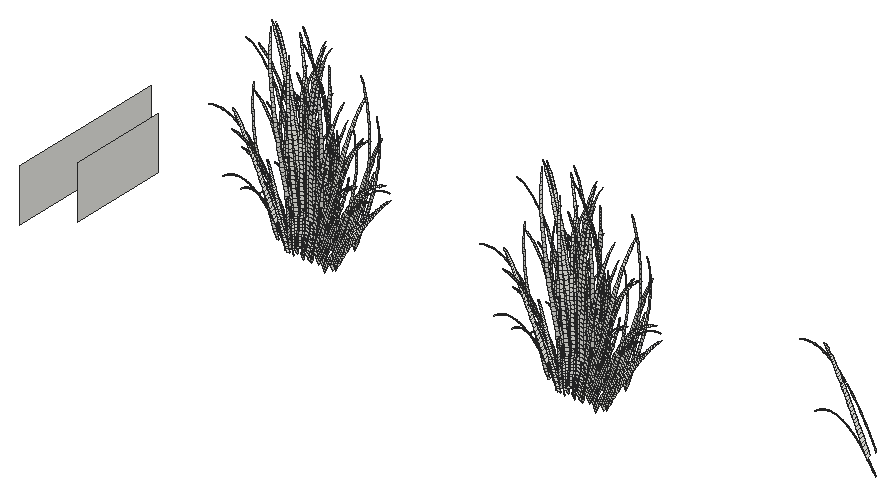
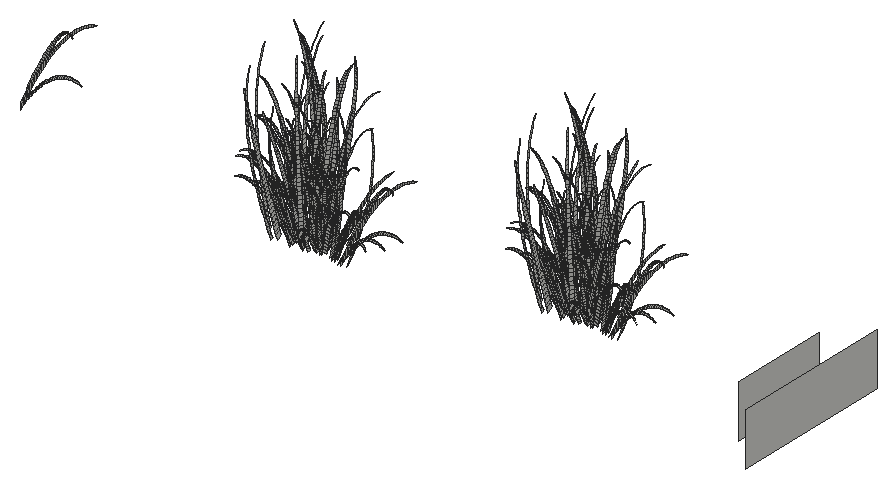
# SketchUp Ruby script. Lengths in inches.
U = 1.inch
M = Sketchup.active_model
def pt(a) = Geom::Point3d.new(a.map { |v| v * U })
def face(e, loops, mat)
  f = e.add_face(loops[0].map { |a| pt(a) })
  loops[1..].each { |l| e.add_face(l.map { |a| pt(a) }).erase! }
  f.material = f.back_material = mat if mat
  f
end
# faces: each face lists its corners as indices into pts; further lists are holes
def faces(e, pts, list, mat = nil) = list.each { |f| face(e, (f[0].is_a?(Array) ? f : [f]).map { |l| l.map { |i| pts[i] } }, mat) }
# xy, xz, yz: faces in a plane at the given z, y or x. An outline is a flat list of corners, or four numbers for a rectangle; further outlines are holes
def ring(l) = l.size == 4 ? [[l[0], l[1]], [l[2], l[1]], [l[2], l[3]], [l[0], l[3]]] : l.each_slice(2).to_a
def flat(e, list, mat, &to3) = list.each { |f| face(e, (f[0].is_a?(Array) ? f : [f]).map { |l| ring(l).map { |u, v| to3.(u, v) } }, mat) }
def xy(e, z, list, mat = nil) = flat(e, list, mat) { |x, y| [x, y, z] }
def xz(e, y, list, mat = nil) = flat(e, list, mat) { |x, z| [x, y, z] }
def yz(e, x, list, mat = nil) = flat(e, list, mat) { |y, z| [x, y, z] }
def lines(e, pts, list) = list.each { |a, b| e.add_line(pt(pts[a]), pt(pts[b])) }
# prism: a flat outline (further loops are holes) pulled along v
def prism(e, loops, v, mat = nil)
  f = face(e, loops, mat); d = Geom::Vector3d.new(v.map { |x| x * U })
  f.pushpull(f.normal.samedirection?(d) ? d.length : -d.length)
end
def box(e, o, s, mat = nil) = prism(e, [[o, [o[0] + s[0], o[1], o[2]], [o[0] + s[0], o[1] + s[1], o[2]], [o[0], o[1] + s[1], o[2]]]], [0, 0, s[2]], mat)
def at(x, y, z, deg = 0) = Geom::Transformation.translation(pt([x, y, z])) * Geom::Transformation.rotation(ORIGIN, Z_AXIS, deg.degrees)
def axes(o, x, y, z) = Geom::Transformation.new([*x, 0, *y, 0, *z, 0, *pt(o).to_a, 1])
def part(name) = M.definitions.add(name)
# library, detail: a bought-in or finely detailed component or shape, given as its bounding box
def library(name, o, s) = part(name).tap { |d| box(d.entities, o, s) }
def detail(e, o, s) = box(e.add_group.entities, o, s)
def put(e, d, t, mat = nil) = e.add_instance(d, t).tap { |i| i.material = mat if mat }
def group(e, t, mat = nil) = e.add_group.tap { |g| g.transformation = t; g.material = mat if mat }.entities
root = M.entities
c1 = part("fur_instance\#8")
p = [[-0.25,1.49,0.03],[0.25,-1.49,-0.03],[0.44,-1.47,1.51],[-0.05,1.47,1.57],[0.65,-1.44,3.05],[0.16,1.45,3.11],
  [0.86,-1.42,4.59],[0.38,1.44,4.65],[1.1,-1.39,6.13],[0.62,1.43,6.18],[1.34,-1.35,7.66],[0.875,1.42,7.72],
  [1.6,-1.32,9.19],[1.14,1.41,9.25],[1.88,-1.28,10.72],[1.43,1.41,10.78],[2.18,-1.24,12.25],[1.73,1.41,12.3],
  [2.49,-1.19,13.77],[2.05,1.41,13.82],[2.83,-1.15,15.29],[2.4,1.41,15.34],[3.18,-1.09,16.8],[2.76,1.42,16.85],
  [3.56,-1.03,18.31],[3.14,1.43,18.35],[3.96,-0.97,19.81],[3.55,1.44,19.85],[4.38,-0.91,21.3],[3.99,1.46,21.35],
  [4.84,-0.83,22.78],[4.45,1.48,22.83],[5.32,-0.76,24.26],[4.93,1.51,24.31],[5.82,-0.67,25.73],[5.45,1.54,25.77],
  [6.36,-0.59,27.18],[6,1.57,27.23],[6.93,-0.49,28.625],[6.58,1.61,28.67],[7.54,-0.39,30.05],[7.19,1.66,30.1],
  [8.18,-0.28,31.47],[7.84,1.71,31.51],[8.85,-0.16,32.86],[8.53,1.77,32.9],[9.57,-0.04,34.24],[9.25,1.83,34.27],
  [10.32,0.09,35.59],[10.02,1.9,35.625],[11.12,0.23,36.92],[10.82,1.97,36.95],[11.95,0.38,38.22],[11.67,2.06,38.25],
  [12.84,0.54,39.49],[12.57,2.14,39.52],[13.76,0.71,40.73],[13.51,2.24,40.76],[14.73,0.89,41.93],[14.49,2.34,41.95],
  [15.75,1.08,43.09],[15.52,2.45,43.11],[16.82,1.28,44.2],[16.6,2.5625,44.23],[17.93,1.5,45.27],[17.73,2.68,45.29],
  [19.08,1.73,46.28],[18.9,2.81,46.3],[20.29,1.97,47.24],[20.125,2.93,47.26],[21.53,2.22,48.13],[21.39,3.0625,48.15],
  [22.82,2.5,48.96],[22.7,3.1875,48.98],[24.14,2.8125,49.72],[24.06,3.3,49.73],[25.48,3.27,50.41]]
faces(c1.entities,p,[[0,1,2,3],[3,2,4,5],[5,4,6,7],[7,6,8,9],[9,8,10,11],[11,10,12,13],[13,12,14,15],[15,14,16,17],
  [17,16,18,19],[19,18,20,21],[21,20,22,23],[23,22,24,25],[25,24,26,27],[27,26,28,29],[29,28,30,31],[31,30,32,33],
  [33,32,34,35],[35,34,36,37],[37,36,38,39],[39,38,40,41],[41,40,42,43],[43,42,44,45],[45,44,46,47],[47,46,48,49],
  [49,48,50,51],[51,50,52,53],[53,52,54,55],[55,54,56,57],[57,56,58,59],[59,58,60,61],[61,60,62,63],[63,62,64,65],
  [65,64,66,67],[67,66,68,69],[69,68,70,71],[71,70,72,73],[73,72,74,75],[75,74,76]])
yz(root,5.25,[[54.02,0,86.15,10.375]])
yz(root,11.52,[[60.29,0,79.88,10.375]])
put(root,c1,axes([46.6,68.06,3.57],[-0.10384,0.1021,-0.23208],[-0.0841,-0.12138,-0.04288],[-0.10059,0.0191,0.29067]))
put(root,c1,axes([99.86,68.06,-2.35],[-0.10384,0.1021,-0.23208],[-0.0841,-0.12138,-0.04288],[-0.10059,0.0191,0.29067]))
put(root,c1,axes([48.45,70.77,6.04],[0.05449,-0.17808,0.19773],[0.18828,0.03949,-0.026],[-0.02035,0.04645,0.39347]))
put(root,c1,axes([101.71,70.77,0.12],[0.05449,-0.17808,0.19773],[0.18828,0.03949,-0.026],[-0.02035,0.04645,0.39347]))
put(root,c1,axes([50.28,68.19,4.32],[-0.15815,0.00988,0.0597],[0.01239,-0.13945,0.21255],[0.01922,0.06125,0.28145]))
put(root,c1,axes([103.54,68.19,-1.59],[-0.15815,0.00988,0.0597],[0.01239,-0.13945,0.21255],[0.01922,0.06125,0.28145]))
put(root,c1,axes([44.41,70.96,4.15],[-0.1218,-0.13361,-0.0921],[0.11484,-0.14709,0.28095],[-0.12602,0.02393,0.36414]))
put(root,c1,axes([97.67,70.96,-1.77],[-0.1218,-0.13361,-0.0921],[0.11484,-0.14709,0.28095],[-0.12602,0.02393,0.36414]))
put(root,c1,axes([50.11,68.81,11.33],[0.06704,0.21243,0.03183],[-0.23851,0.07708,0.05394],[0.01333,-0.07138,0.55186]))
put(root,c1,axes([103.37,68.81,5.41],[0.06704,0.21243,0.03183],[-0.23851,0.07708,0.05394],[0.01333,-0.07138,0.55186]))
put(root,c1,axes([52.26,71.8,10.58],[-0.21942,-0.09635,0.15751],[0.11362,-0.22061,0.00466],[0.05601,-0.02476,0.54483]))
put(root,c1,axes([105.51,71.8,4.66],[-0.21942,-0.09635,0.15751],[0.11362,-0.22061,0.00466],[0.05601,-0.02476,0.54483]))
put(root,c1,axes([45.97,69.1,10.95],[-0.01349,0.22403,0.09768],[-0.24396,0.034,-0.14422],[-0.06912,-0.0865,0.54108]))
put(root,c1,axes([99.23,69.1,5.03],[-0.01349,0.22403,0.09768],[-0.24396,0.034,-0.14422],[-0.06912,-0.0865,0.54108]))
put(root,c1,axes([50.68,68.57,9.98],[0.01128,0.21113,0.01155],[-0.2291,0.02553,0.05014],[0.01651,-0.05502,0.51224]))
put(root,c1,axes([103.9375,68.57,4.07],[0.01128,0.21113,0.01155],[-0.2291,0.02553,0.05014],[0.01651,-0.05502,0.51224]))
put(root,c1,axes([51.88,69.84,2.47],[-0.03747,-0.12843,0.29203],[0.15407,-0.08219,-0.0652],[0.07562,0.07004,0.25518]))
put(root,c1,axes([105.14,69.84,-3.45],[-0.03747,-0.12843,0.29203],[0.15407,-0.08219,-0.0652],[0.07562,0.07004,0.25518]))
put(root,c1,axes([47.78,68.6875,10],[-0.05249,0.21081,0.00883],[-0.2212,-0.0235,-0.05439],[-0.02833,-0.05377,0.50988]))
put(root,c1,axes([101.04,68.6875,4.08],[-0.05249,0.21081,0.00883],[-0.2212,-0.0235,-0.05439],[-0.02833,-0.05377,0.50988]))
put(root,c1,axes([47.3,67.75,4.56],[0.05338,0.14377,-0.04693],[-0.14103,0.06373,-0.16463],[-0.0677,0.01402,0.32804]))
put(root,c1,axes([100.5625,67.75,-1.36],[0.05338,0.14377,-0.04693],[-0.14103,0.06373,-0.16463],[-0.0677,0.01402,0.32804]))
put(root,c1,axes([49.55,69.22,11.72],[0.09204,0.20501,0.03679],[-0.23374,0.09978,0.05402],[0.01033,-0.07544,0.55902]))
put(root,c1,axes([102.8125,69.22,5.8],[0.09204,0.20501,0.03679],[-0.23374,0.09978,0.05402],[0.01033,-0.07544,0.55902]))
put(root,c1,axes([51.37,68.6,8.54],[0.05117,0.19348,-0.04619],[-0.20175,0.05612,0.13032],[0.05644,-0.043,0.46253]))
put(root,c1,axes([104.625,68.6,2.625],[0.05117,0.19348,-0.04619],[-0.20175,0.05612,0.13032],[0.05644,-0.043,0.46253]))
put(root,c1,axes([46.68,69.78,8.34],[-0.20159,0.0718,-0.13723],[-0.04865,-0.19336,0.01671],[-0.06325,-0.01861,0.46524]))
put(root,c1,axes([99.94,69.78,2.42],[-0.20159,0.0718,-0.13723],[-0.04865,-0.19336,0.01671],[-0.06325,-0.01861,0.46524]))
put(root,c1,axes([48.14,68.42,5],[0.14782,0.0607,0.01728],[-0.06736,0.14608,-0.17165],[-0.04658,0.03213,0.33667]))
put(root,c1,axes([101.4,68.42,-0.92],[0.14782,0.0607,0.01728],[-0.06736,0.14608,-0.17165],[-0.04658,0.03213,0.33667]))
put(root,c1,axes([46.58,69.4,2.61],[-0.13656,-0.07352,-0.06681],[0.04427,-0.12761,0.28622],[-0.09439,0.0724,0.24805]))
put(root,c1,axes([99.84,69.4,-3.3125],[-0.13656,-0.07352,-0.06681],[0.04427,-0.12761,0.28622],[-0.09439,0.0724,0.24805]))
put(root,c1,axes([50.73,67.71,4.39],[-0.04536,0.14528,-0.12173],[-0.14819,-0.02558,0.10276],[0.0266,0.02828,0.3139]))
put(root,c1,axes([103.99,67.71,-1.53],[-0.04536,0.14528,-0.12173],[-0.14819,-0.02558,0.10276],[0.0266,0.02828,0.3139]))
put(root,c1,axes([49.54,69.48,6.28],[0.18587,-0.039,0.02017],[0.0261,0.16941,-0.18858],[-0.00202,0.04384,0.37494]))
put(root,c1,axes([102.79,69.48,0.36],[0.18587,-0.039,0.02017],[0.0261,0.16941,-0.18858],[-0.00202,0.04384,0.37494]))
put(root,c1,axes([48.4,68.13,4.75],[-0.10713,0.11469,-0.16211],[-0.11423,-0.10051,0.03718],[-0.0449,0.03097,0.32456]))
put(root,c1,axes([101.65,68.13,-1.17],[-0.10713,0.11469,-0.16211],[-0.11423,-0.10051,0.03718],[-0.0449,0.03097,0.32456]))
put(root,c1,axes([48.33,71.86,12.25],[0.25389,-0.06297,0.01758],[0.0429,0.23535,-0.03956],[-0.01113,-0.0353,0.57531]))
put(root,c1,axes([101.59,71.86,6.33],[0.25389,-0.06297,0.01758],[0.0429,0.23535,-0.03956],[-0.01113,-0.0353,0.57531]))
put(root,c1,axes([50.25,69.88,8.7],[-0.20845,0.0617,0.05447],[-0.04632,-0.1966,0.1192],[0.03082,-0.00313,0.46484]))
put(root,c1,axes([103.5,69.88,2.78],[-0.20845,0.0617,0.05447],[-0.04632,-0.1966,0.1192],[0.03082,-0.00313,0.46484]))
put(root,c1,axes([47.47,69.95,3.72],[0.12753,-0.09379,0.22491],[0.10527,0.1265,-0.10063],[-0.06372,0.06207,0.3109]))
put(root,c1,axes([100.73,69.95,-2.2],[0.12753,-0.09379,0.22491],[0.10527,0.1265,-0.10063],[-0.06372,0.06207,0.3109]))
put(root,c1,axes([45.17,70.53,3.39],[-0.12578,-0.12091,-0.0564],[0.08033,-0.12818,0.33188],[-0.12725,0.06361,0.28183]))
put(root,c1,axes([98.43,70.53,-2.53],[-0.12578,-0.12091,-0.0564],[0.08033,-0.12818,0.33188],[-0.12725,0.06361,0.28183]))
put(root,c1,axes([47.78,68.82,3.42],[0.15191,0.00864,0.09894],[-0.00116,0.14441,-0.20359],[-0.05853,0.05702,0.28561]))
put(root,c1,axes([101.04,68.82,-2.49],[0.15191,0.00864,0.09894],[-0.00116,0.14441,-0.20359],[-0.05853,0.05702,0.28561]))
put(root,c1,axes([53.59,68.1,2.85],[0.00579,0.17068,-0.16321],[-0.12957,0.03754,0.26919],[0.12935,0.00849,0.26276]))
put(root,c1,axes([106.85,68.1,-3.07],[0.00579,0.17068,-0.16321],[-0.12957,0.03754,0.26919],[0.12935,0.00849,0.26276]))
put(root,c1,axes([47.39,69,3.82],[0.15072,0.0136,0.13727],[-0.00409,0.15385,-0.193],[-0.07769,0.04892,0.29677]))
put(root,c1,axes([100.65,69,-2.1],[0.15072,0.0136,0.13727],[-0.00409,0.15385,-0.193],[-0.07769,0.04892,0.29677]))
put(root,c1,axes([49.1,69.77,3.04],[-0.01699,-0.12732,0.27857],[0.16448,-0.01291,0.05595],[-0.02464,0.09551,0.24356]))
put(root,c1,axes([102.36,69.77,-2.88],[-0.01699,-0.12732,0.27857],[0.16448,-0.01291,0.05595],[-0.02464,0.09551,0.24356]))
put(root,c1,axes([46.98,71.28,8.64],[0.21265,-0.06804,0.11906],[0.05038,0.20319,-0.07151],[-0.05071,-0.00134,0.48262]))
put(root,c1,axes([100.24,71.28,2.72],[0.21265,-0.06804,0.11906],[0.05038,0.20319,-0.07151],[-0.05071,-0.00134,0.48262]))
put(root,c1,axes([52.3125,69.17,4.93],[-0.16864,0.05731,0.14747],[-0.02228,-0.16808,0.21885],[0.0836,0.03526,0.33224]))
put(root,c1,axes([105.57,69.17,-0.99],[-0.16864,0.05731,0.14747],[-0.02228,-0.16808,0.21885],[0.0836,0.03526,0.33224]))
put(root,c1,axes([51.91,70.15,3.16],[0.14782,-0.11273,0.00048],[0.0732,0.11159,-0.31128],[0.07867,0.07287,0.26546]))
put(root,c1,axes([105.17,70.15,-2.76],[0.14782,-0.11273,0.00048],[0.0732,0.11159,-0.31128],[0.07867,0.07287,0.26546]))
put(root,c1,axes([43.62,70.74,3.37],[-0.13408,-0.01944,-0.33055],[0.01755,-0.20151,0.16145],[-0.16419,0.01714,0.30229]))
put(root,c1,axes([96.88,70.74,-2.55],[-0.13408,-0.01944,-0.33055],[0.01755,-0.20151,0.16145],[-0.16419,0.01714,0.30229]))
put(root,c1,axes([159.93,70.74,2.83],[-0.13408,-0.01944,-0.33055],[0.01755,-0.20151,0.16145],[-0.16419,0.01714,0.30229]))
put(root,c1,axes([42.5,70.72,3.15],[0.14067,-0.04522,0.3848],[0.02544,0.20918,-0.05629],[-0.17357,0.01812,0.31957]))
put(root,c1,axes([95.76,70.72,-2.77],[0.14067,-0.04522,0.3848],[0.02544,0.20918,-0.05629],[-0.17357,0.01812,0.31957]))
put(root,c1,axes([44.92,69.8,2.44],[-0.1289,0.01316,-0.29885],[-0.02366,-0.17656,0.13341],[-0.13753,0.03975,0.27153]))
put(root,c1,axes([98.18,69.8,-3.48],[-0.1289,0.01316,-0.29885],[-0.02366,-0.17656,0.13341],[-0.13753,0.03975,0.27153]))
put(root,c1,axes([50.5625,70.22,2.63],[0.01055,-0.13508,0.28615],[0.17058,-0.02073,-0.06684],[0.02674,0.09288,0.2522]))
put(root,c1,axes([103.82,70.22,-3.29],[0.01055,-0.13508,0.28615],[0.17058,-0.02073,-0.06684],[0.02674,0.09288,0.2522]))
put(root,c1,axes([52.4,68.97,7.36],[0.08157,0.17825,-0.15725],[-0.17491,0.09532,0.15482],[0.08885,-0.01806,0.42132]))
put(root,c1,axes([105.66,68.97,1.4375],[0.08157,0.17825,-0.15725],[-0.17491,0.09532,0.15482],[0.08885,-0.01806,0.42132]))
put(root,c1,axes([47.85,69.31,4.49],[0.16194,-0.0082,0.12991],[0.01706,0.15486,-0.20493],[-0.06274,0.06113,0.30616]))
put(root,c1,axes([101.11,69.31,-1.43],[0.16194,-0.0082,0.12991],[0.01706,0.15486,-0.20493],[-0.06274,0.06113,0.30616]))
put(root,c1,axes([49.32,69.43,8.14],[-0.17716,0.11278,-0.05906],[-0.10338,-0.15992,0.10796],[-0.00363,0.01008,0.44244]))
put(root,c1,axes([102.58,69.43,2.22],[-0.17716,0.11278,-0.05906],[-0.10338,-0.15992,0.10796],[-0.00363,0.01008,0.44244]))
put(root,c1,axes([48.89,68.12,5.35],[0.03769,0.14922,-0.14278],[-0.15939,0.04231,-0.09138],[-0.03216,0.03689,0.33298]))
put(root,c1,axes([102.15,68.12,-0.57],[0.03769,0.14922,-0.14278],[-0.15939,0.04231,-0.09138],[-0.03216,0.03689,0.33298]))
put(root,c1,axes([49.02,68.34,4.09],[0.13054,0.07134,-0.09742],[-0.08675,0.11604,-0.1956],[-0.0202,0.06504,0.27821]))
put(root,c1,axes([102.28,68.34,-1.83],[0.13054,0.07134,-0.09742],[-0.08675,0.11604,-0.1956],[-0.0202,0.06504,0.27821]))
put(root,c1,axes([45.96,69.02,2.9],[-0.11086,0.06293,-0.29386],[-0.07533,-0.1452,0.07106],[-0.11428,0.05713,0.25311]))
put(root,c1,axes([99.22,69.02,-3.02],[-0.11086,0.06293,-0.29386],[-0.07533,-0.1452,0.07106],[-0.11428,0.05713,0.25311]))
put(root,c1,axes([51.5625,71.14,4.15],[-0.10724,-0.12303,0.26265],[0.15657,-0.12402,0.06415],[0.04661,0.06574,0.34387]))
put(root,c1,axes([104.82,71.14,-1.77],[-0.10724,-0.12303,0.26265],[0.15657,-0.12402,0.06415],[0.04661,0.06574,0.34387]))
put(root,c1,axes([50.5,68.99,2.82],[-0.15615,0.01011,0.08042],[0.021,-0.12557,0.25868],[0.02465,0.08562,0.2325]))
put(root,c1,axes([103.76,68.99,-3.1],[-0.15615,0.01011,0.08042],[0.021,-0.12557,0.25868],[0.02465,0.08562,0.2325]))
put(root,c1,axes([45.83,70.21,2.8],[0.12181,-0.05572,0.30355],[0.07119,0.15699,-0.09562],[-0.1203,0.06014,0.26644]))
put(root,c1,axes([99.09,70.21,-3.12],[0.12181,-0.05572,0.30355],[0.07119,0.15699,-0.09562],[-0.1203,0.06014,0.26644]))
put(root,c1,axes([50.5,69.51,6.67],[-0.18299,0.07424,0.021],[-0.05602,-0.16634,0.19558],[0.03285,0.03492,0.38761]))
put(root,c1,axes([103.76,69.51,0.75],[-0.18299,0.07424,0.021],[-0.05602,-0.16634,0.19558],[0.03285,0.03492,0.38761]))
put(root,c1,axes([48.49,69.36,9.71],[-0.02533,0.21082,-0.03246],[-0.22123,-0.00286,-0.02372],[-0.01766,-0.03271,0.49841]))
put(root,c1,axes([101.75,69.36,3.79],[-0.02533,0.21082,-0.03246],[-0.22123,-0.00286,-0.02372],[-0.01766,-0.03271,0.49841]))
put(root,c1,axes([50.65,71.25,11.53],[-0.23935,0.06874,0.11641],[-0.05487,-0.22915,0.10476],[0.05566,-0.0246,0.54145]))
put(root,c1,axes([103.91,71.25,5.61],[-0.23935,0.06874,0.11641],[-0.05487,-0.22915,0.10476],[0.05566,-0.0246,0.54145]))
put(root,c1,axes([49.7,68.87,7.19],[-0.04271,0.18174,-0.10347],[-0.18723,-0.02484,0.051],[0.00749,0.00721,0.41447]))
put(root,c1,axes([102.96,68.87,1.27],[-0.04271,0.18174,-0.10347],[-0.18723,-0.02484,0.051],[0.00749,0.00721,0.41447]))
put(root,c1,axes([45.79,68.9,4.06],[-0.0676,0.15738,-0.2157],[-0.13135,-0.07732,-0.14677],[-0.1112,0.02111,0.32133]))
put(root,c1,axes([99.05,68.9,-1.85],[-0.0676,0.15738,-0.2157],[-0.13135,-0.07732,-0.14677],[-0.1112,0.02111,0.32133]))
put(root,c1,axes([48.63,69.14,2.66],[-0.14803,0.01323,-0.11537],[-0.03176,-0.12328,0.24366],[-0.04653,0.08668,0.23028]))
put(root,c1,axes([101.89,69.14,-3.26],[-0.14803,0.01323,-0.11537],[-0.03176,-0.12328,0.24366],[-0.04653,0.08668,0.23028]))
put(root,c1,axes([53.61,69.47,3.23],[-0.14434,0.09377,0.17872],[-0.03919,-0.15638,0.28066],[0.124,0.03453,0.28007]))
put(root,c1,axes([106.87,69.47,-2.69],[-0.14434,0.09377,0.17872],[-0.03919,-0.15638,0.28066],[0.124,0.03453,0.28007]))
put(root,c1,axes([53.2,69.52,5.76],[0.1044,0.14559,-0.25751],[-0.13502,0.13555,0.13946],[0.11942,-0.00409,0.36287]))
put(root,c1,axes([106.46,69.52,-0.16],[0.1044,0.14559,-0.25751],[-0.13502,0.13555,0.13946],[0.11942,-0.00409,0.36287]))
put(root,c1,axes([52.8,69.59,9.125],[0.01228,0.22259,-0.04839],[-0.21245,0.01489,0.2439],[0.10506,-0.04029,0.46949]))
put(root,c1,axes([106.06,69.59,3.21],[0.01228,0.22259,-0.04839],[-0.21245,0.01489,0.2439],[0.10506,-0.04029,0.46949]))
put(root,c1,axes([48.66,70.2,3.2],[0.1046,-0.10479,0.24905],[0.1356,0.08115,-0.15676],[-0.02552,0.09892,0.25225]))
put(root,c1,axes([101.92,70.2,-2.72],[0.1046,-0.10479,0.24905],[0.1356,0.08115,-0.15676],[-0.02552,0.09892,0.25225]))
put(root,c1,axes([52.125,69.5625,4.6],[-0.15929,0.09132,0.09708],[-0.05737,-0.15132,0.24406],[0.08321,0.03509,0.33068]))
put(root,c1,axes([105.38,69.5625,-1.32],[-0.15929,0.09132,0.09708],[-0.05737,-0.15132,0.24406],[0.08321,0.03509,0.33068]))
put(root,c1,axes([45.73,72.36,4.95],[0.01665,-0.19186,0.25247],[0.18867,0.0288,0.15737],[-0.09759,0.06145,0.3728]))
put(root,c1,axes([98.99,72.36,-0.97],[0.01665,-0.19186,0.25247],[0.18867,0.0288,0.15737],[-0.09759,0.06145,0.3728]))
put(root,c1,axes([51.63,69.15,3.2],[-0.15229,0.06835,0.08842],[-0.02287,-0.13137,0.27682],[0.07344,0.06802,0.24782]))
put(root,c1,axes([104.89,69.15,-2.72],[-0.15229,0.06835,0.08842],[-0.02287,-0.13137,0.27682],[0.07344,0.06802,0.24782]))
put(root,c1,axes([51.95,68.76,3.32],[-0.11038,0.13094,-0.01587],[-0.09023,-0.08182,0.28993],[0.09271,0.05046,0.24619]))
put(root,c1,axes([105.21,68.76,-2.6],[-0.11038,0.13094,-0.01587],[-0.09023,-0.08182,0.28993],[0.09271,0.05046,0.24619]))
put(root,c1,axes([50.46,69.33,4.24],[0.1552,0.04284,-0.14088],[-0.07244,0.14474,-0.19228],[0.02075,0.06614,0.30388]))
put(root,c1,axes([103.72,69.33,-1.68],[0.1552,0.04284,-0.14088],[-0.07244,0.14474,-0.19228],[0.02075,0.06614,0.30388]))
put(root,c1,axes([47.2,70.96,12.28],[-0.19599,0.17659,-0.04249],[-0.16606,-0.16516,-0.03794],[-0.03174,-0.0516,0.57661]))
put(root,c1,axes([100.46,70.96,6.36],[-0.19599,0.17659,-0.04249],[-0.16606,-0.16516,-0.03794],[-0.03174,-0.0516,0.57661]))
put(root,c1,axes([48.41,70.02,8.49],[0.1688,0.10784,-0.0329],[-0.12628,0.17185,-0.12449],[-0.0276,0.0088,0.45819]))
put(root,c1,axes([101.67,70.02,2.57],[0.1688,0.10784,-0.0329],[-0.12628,0.17185,-0.12449],[-0.0276,0.0088,0.45819]))
put(root,c1,axes([54.09,69.51,2.62],[-0.08133,0.16944,0.041],[-0.11353,-0.08181,0.33645],[0.13926,0.00914,0.28291]))
put(root,c1,axes([107.35,69.51,-3.3],[-0.08133,0.16944,0.041],[-0.11353,-0.08181,0.33645],[0.13926,0.00914,0.28291]))
put(root,c1,axes([45.2,70.27,7.74],[0.12687,0.1431,0.11306],[-0.15006,0.15928,-0.20805],[-0.10892,-0.0144,0.44372]))
put(root,c1,axes([98.45,70.27,1.82],[0.12687,0.1431,0.11306],[-0.15006,0.15928,-0.20805],[-0.10892,-0.0144,0.44372]))
put(root,c1,axes([47.35,68.76,3.7],[-0.00457,0.15131,-0.19037],[-0.14827,-0.01393,-0.13436],[-0.07643,0.04813,0.29198]))
put(root,c1,axes([100.61,68.76,-2.22],[-0.00457,0.15131,-0.19037],[-0.14827,-0.01393,-0.13436],[-0.07643,0.04813,0.29198]))
put(root,c1,axes([45.06,71.55,4.26],[0.1591,-0.07433,0.27972],[0.07325,0.17912,-0.08368],[-0.11229,0.04342,0.36287]))
put(root,c1,axes([98.32,71.55,-1.66],[0.1591,-0.07433,0.27972],[0.07325,0.17912,-0.08368],[-0.11229,0.04342,0.36287]))
put(root,c1,axes([51.04,70.95,7.6],[0.2064,0.00506,-0.149],[-0.0314,0.20396,-0.16093],[0.05385,0.02809,0.42994]))
put(root,c1,axes([104.3,70.95,1.68],[0.2064,0.00506,-0.149],[-0.0314,0.20396,-0.16093],[0.05385,0.02809,0.42994]))
put(root,c1,axes([51.12,69.43,5.23],[-0.1523,0.1081,0.01181],[-0.08113,-0.12936,0.25496],[0.06382,0.04964,0.32324]))
put(root,c1,axes([104.375,69.43,-0.69],[-0.1523,0.1081,0.01181],[-0.08113,-0.12936,0.25496],[0.06382,0.04964,0.32324]))
put(root,c1,axes([47.76,70.72,3.61],[0.16515,-0.05448,0.15409],[0.06343,0.14946,-0.20076],[-0.0453,0.07156,0.32105]))
put(root,c1,axes([101.02,70.72,-2.31],[0.16515,-0.05448,0.15409],[0.06343,0.14946,-0.20076],[-0.0453,0.07156,0.32105]))
put(root,c1,axes([47.05,69.79,4.01],[-0.13323,0.08202,-0.23675],[-0.08835,-0.14174,0.08371],[-0.08237,0.05187,0.31467]))
put(root,c1,axes([100.31,69.79,-1.91],[-0.13323,0.08202,-0.23675],[-0.08835,-0.14174,0.08371],[-0.08237,0.05187,0.31467]))
put(root,c1,axes([50.83,71.84,5.96],[0.16589,-0.13509,0.0734],[0.11769,0.12965,-0.28034],[0.04996,0.07046,0.36857]))
put(root,c1,axes([104.09,71.84,0.04],[0.16589,-0.13509,0.0734],[0.11769,0.12965,-0.28034],[0.04996,0.07046,0.36857]))
put(root,c1,axes([53.09,70.89,4.85],[0.18376,0.00291,-0.23488],[-0.03958,0.19621,-0.17283],[0.09238,0.03896,0.36714]))
put(root,c1,axes([106.35,70.89,-1.07],[0.18376,0.00291,-0.23488],[-0.03958,0.19621,-0.17283],[0.09238,0.03896,0.36714]))
put(root,c1,axes([52.1875,70.99,4.27],[0.18658,-0.03164,-0.14855],[-0.00603,0.17961,-0.23275],[0.06904,0.0537,0.34969]))
put(root,c1,axes([105.44,70.99,-1.65],[0.18658,-0.03164,-0.14855],[-0.00603,0.17961,-0.23275],[0.06904,0.0537,0.34969]))
put(root,c1,axes([53.26,71.46,3.26],[-0.14001,-0.05504,0.33454],[0.10116,-0.17879,0.10883],[0.11232,0.06113,0.29828]))
put(root,c1,axes([106.52,71.46,-2.66],[-0.14001,-0.05504,0.33454],[0.10116,-0.17879,0.10883],[0.11232,0.06113,0.29828]))
put(root,c1,axes([42.59,70.33,6.35],[-0.11905,0.20326,-0.22454],[-0.13951,-0.10936,-0.26462],[-0.15957,-0.02537,0.41917]))
put(root,c1,axes([95.85,70.33,0.43],[-0.11905,0.20326,-0.22454],[-0.13951,-0.10936,-0.26462],[-0.15957,-0.02537,0.41917]))
put(root,c1,axes([158.9,70.33,5.8],[-0.11905,0.20326,-0.22454],[-0.13951,-0.10936,-0.26462],[-0.15957,-0.02537,0.41917]))
put(root,c1,axes([45.48,72.79,11.08],[-0.24661,-0.01011,-0.12308],[0.03558,-0.24626,0.10561],[-0.06805,-0.01098,0.55498]))
put(root,c1,axes([98.74,72.79,5.16],[-0.24661,-0.01011,-0.12308],[0.03558,-0.24626,0.10561],[-0.06805,-0.01098,0.55498]))
put(root,c1,axes([56.15,72.8,5.625],[-0.20751,-0.0154,0.34807],[0.03231,-0.24429,0.09326],[0.14695,-0.00503,0.44651]))
put(root,c1,axes([109.41,72.8,-0.3],[-0.20751,-0.0154,0.34807],[0.03231,-0.24429,0.09326],[0.14695,-0.00503,0.44651]))
put(root,c1,axes([49.43,73.46,8.17],[0.08686,-0.20683,0.21585],[0.21659,0.06277,-0.09493],[-0.00252,0.05451,0.46618]))
put(root,c1,axes([102.6875,73.46,2.25],[0.08686,-0.20683,0.21585],[0.21659,0.06277,-0.09493],[-0.00252,0.05451,0.46618]))
put(root,c1,axes([47.2,71.36,12.11],[-0.19695,0.1732,-0.04859],[-0.16287,-0.16855,-0.01576],[-0.02749,-0.04327,0.57313]))
put(root,c1,axes([100.46,71.36,6.19],[-0.19695,0.1732,-0.04859],[-0.16287,-0.16855,-0.01576],[-0.02749,-0.04327,0.57313]))
put(root,c1,axes([45.88,70.27,3.32],[0.14298,0.02776,0.2221],[0.00324,0.16655,-0.23396],[-0.12194,0.06096,0.27007]))
put(root,c1,axes([99.14,70.27,-2.6],[0.14298,0.02776,0.2221],[0.00324,0.16655,-0.23396],[-0.12194,0.06096,0.27007]))
put(root,c1,axes([41.27,73.83,5.51],[-0.16665,-0.10839,-0.24928],[0.10528,-0.22,0.26583],[-0.16455,0.00217,0.44452]))
put(root,c1,axes([94.53,73.83,-0.41],[-0.16665,-0.10839,-0.24928],[0.10528,-0.22,0.26583],[-0.16455,0.00217,0.44452]))
put(root,c1,axes([157.58,73.83,4.96],[-0.16665,-0.10839,-0.24928],[0.10528,-0.22,0.26583],[-0.16455,0.00217,0.44452]))
put(root,c1,axes([50.25,71.14,5.98],[-0.20063,0.02155,0.04243],[-0.00141,-0.18611,0.19899],[0.01635,0.04322,0.40207]))
put(root,c1,axes([103.51,71.14,0.06],[-0.20063,0.02155,0.04243],[-0.00141,-0.18611,0.19899],[0.01635,0.04322,0.40207]))
put(root,c1,axes([55.1,73.69,4.74],[-0.06693,-0.18459,0.37403],[0.17622,-0.13687,-0.1896],[0.15627,0.04352,0.35297]))
put(root,c1,axes([108.36,73.69,-1.18],[-0.06693,-0.18459,0.37403],[0.17622,-0.13687,-0.1896],[0.15627,0.04352,0.35297]))
put(root,c1,axes([49.7,71.73,5.55],[0.16091,-0.11894,0.16216],[0.12315,0.12828,-0.22813],[-0.0007,0.08282,0.35694]))
put(root,c1,axes([102.96,71.73,-0.37],[0.16091,-0.11894,0.16216],[0.12315,0.12828,-0.22813],[-0.0007,0.08282,0.35694]))
put(root,c1,axes([54.34,69.79,2.75],[-0.00334,0.19157,-0.16025],[-0.14373,0.02868,0.30995],[0.14337,0.00941,0.29124]))
put(root,c1,axes([107.6,69.79,-3.17],[-0.00334,0.19157,-0.16025],[-0.14373,0.02868,0.30995],[0.14337,0.00941,0.29124]))
put(root,c1,axes([51.49,71.38,6.88],[-0.20765,0.04551,0.10452],[-0.02061,-0.19877,0.19268],[0.05382,0.02807,0.42972]))
put(root,c1,axes([104.75,71.38,0.96],[-0.20765,0.04551,0.10452],[-0.02061,-0.19877,0.19268],[0.05382,0.02807,0.42972]))
put(root,c1,axes([53.42,73.91,5.7],[0.12626,-0.20284,0.07113],[0.17291,0.09387,-0.32445],[0.10522,0.04438,0.41818]))
put(root,c1,axes([106.68,73.91,-0.22],[0.12626,-0.20284,0.07113],[0.17291,0.09387,-0.32445],[0.10522,0.04438,0.41818]))
put(root,c1,axes([51.05,69.23,4.14],[0.03504,0.14333,-0.23786],[-0.16522,0.06024,0.03644],[0.04149,0.05851,0.30605]))
put(root,c1,axes([104.3,69.23,-1.78],[0.03504,0.14333,-0.23786],[-0.16522,0.06024,0.03644],[0.04149,0.05851,0.30605]))
put(root,c1,axes([47.78,69.57,4.46],[0.12802,0.10582,-0.05497],[-0.1046,0.11656,-0.24012],[-0.0637,0.06206,0.31081]))
put(root,c1,axes([101.04,69.57,-1.46],[0.12802,0.10582,-0.05497],[-0.1046,0.11656,-0.24012],[-0.0637,0.06206,0.31081]))
put(root,c1,axes([49.24,71.39,6.39],[-0.2047,0.01723,0.00593],[-0.00087,-0.18882,0.20676],[-0.00221,0.04782,0.40893]))
put(root,c1,axes([102.5,71.39,0.47],[-0.2047,0.01723,0.00593],[-0.00087,-0.18882,0.20676],[-0.00221,0.04782,0.40893]))
put(root,c1,axes([47.93,69.89,5.75],[-0.11141,0.14453,-0.18255],[-0.14786,-0.09923,0.0582],[-0.03635,0.0417,0.37637]))
put(root,c1,axes([101.1875,69.89,-0.17],[-0.11141,0.14453,-0.18255],[-0.14786,-0.09923,0.0582],[-0.03635,0.0417,0.37637]))
put(root,c1,axes([51.18,70.18,4.79],[-0.17132,0.08809,0.00001],[-0.06467,-0.14373,0.26091],[0.04498,0.06344,0.33183]))
put(root,c1,axes([104.44,70.18,-1.13],[-0.17132,0.08809,0.00001],[-0.06467,-0.14373,0.26091],[0.04498,0.06344,0.33183]))
put(root,c1,axes([51.24,70.75,3.09],[-0.16842,0.00001,0.17613],[0.0504,-0.15213,0.25899],[0.055,0.08838,0.2682]))
put(root,c1,axes([104.5,70.75,-2.83],[-0.16842,0.00001,0.17613],[0.0504,-0.15213,0.25899],[0.055,0.08838,0.2682]))
put(root,c1,axes([48.35,70.98,4.15],[-0.18524,0.01318,-0.044],[-0.00864,-0.16062,0.25477],[-0.0239,0.07696,0.32915]))
put(root,c1,axes([101.61,70.98,-1.77],[-0.18524,0.01318,-0.044],[-0.00864,-0.16062,0.25477],[-0.0239,0.07696,0.32915]))
put(root,c1,axes([48.91,71.5,11.35],[-0.15522,0.19417,-0.03161],[-0.19201,-0.12962,0.02598],[-0.00591,-0.03393,0.55136]))
put(root,c1,axes([102.17,71.5,5.43],[-0.15522,0.19417,-0.03161],[-0.19201,-0.12962,0.02598],[-0.00591,-0.03393,0.55136]))
put(root,c1,axes([49.86,69.3,2.64],[-0.06121,0.11818,-0.24749],[-0.14799,-0.03414,0.11286],[0.00064,0.09094,0.23354]))
put(root,c1,axes([103.12,69.3,-3.28],[-0.06121,0.11818,-0.24749],[-0.14799,-0.03414,0.11286],[0.00064,0.09094,0.23354]))
put(root,c1,axes([46.01,71.08,7.39],[-0.16212,0.13096,-0.2268],[-0.11678,-0.16208,0.00347],[-0.08971,0.01858,0.43465]))
put(root,c1,axes([99.27,71.08,1.47],[-0.16212,0.13096,-0.2268],[-0.11678,-0.16208,0.00347],[-0.08971,0.01858,0.43465]))
put(root,c1,axes([47.65,70.36,8.72],[0.03814,0.2015,-0.09604],[-0.21147,0.05412,-0.09289],[-0.03952,0.00488,0.47049]))
put(root,c1,axes([100.91,70.36,2.8],[0.03814,0.2015,-0.09604],[-0.21147,0.05412,-0.09289],[-0.03952,0.00488,0.47049]))
put(root,c1,axes([45.11,74.84,8.22],[-0.12046,-0.19753,0.07695],[0.20061,-0.12871,0.24478],[-0.08711,0.03599,0.49657]))
